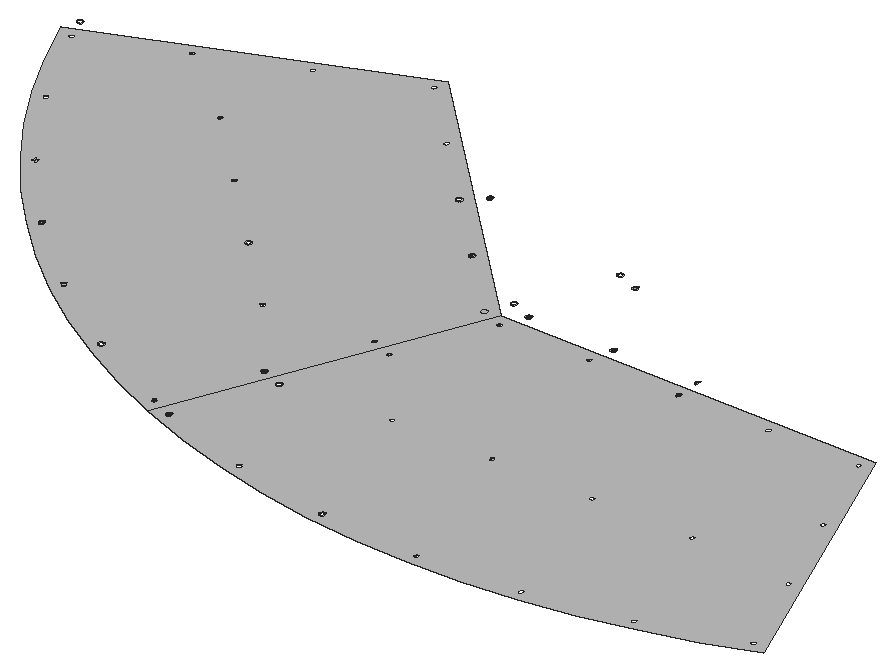
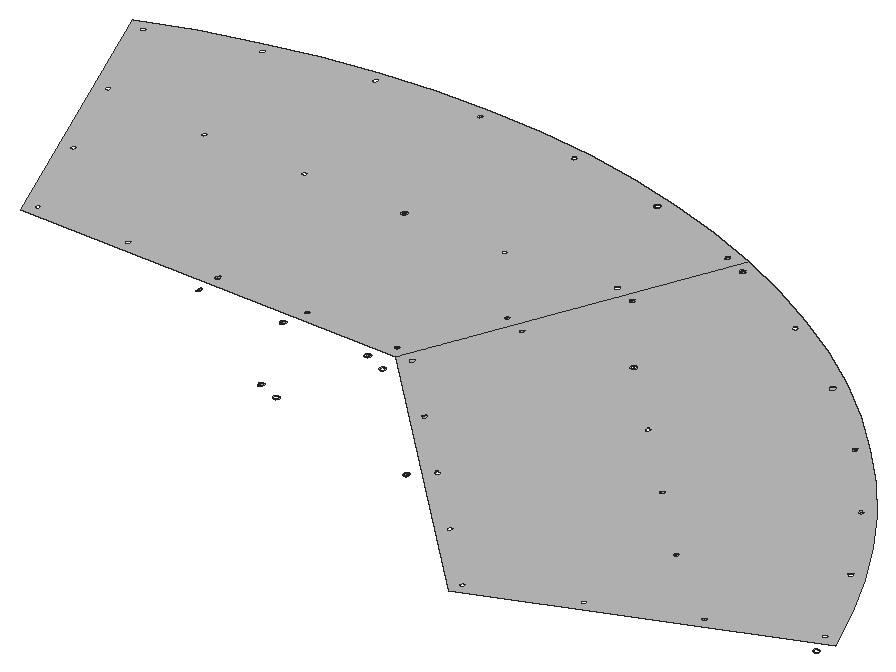
# SketchUp Ruby script. Lengths in inches.
U = 1.inch
M = Sketchup.active_model
def pt(a) = Geom::Point3d.new(a.map { |v| v * U })
def face(e, loops, mat)
  f = e.add_face(loops[0].map { |a| pt(a) })
  loops[1..].each { |l| e.add_face(l.map { |a| pt(a) }).erase! }
  f.material = f.back_material = mat if mat
  f
end
# faces: each face lists its corners as indices into pts; further lists are holes
def faces(e, pts, list, mat = nil) = list.each { |f| face(e, (f[0].is_a?(Array) ? f : [f]).map { |l| l.map { |i| pts[i] } }, mat) }
# xy, xz, yz: faces in a plane at the given z, y or x. An outline is a flat list of corners, or four numbers for a rectangle; further outlines are holes
def ring(l) = l.size == 4 ? [[l[0], l[1]], [l[2], l[1]], [l[2], l[3]], [l[0], l[3]]] : l.each_slice(2).to_a
def flat(e, list, mat, &to3) = list.each { |f| face(e, (f[0].is_a?(Array) ? f : [f]).map { |l| ring(l).map { |u, v| to3.(u, v) } }, mat) }
def xy(e, z, list, mat = nil) = flat(e, list, mat) { |x, y| [x, y, z] }
def xz(e, y, list, mat = nil) = flat(e, list, mat) { |x, z| [x, y, z] }
def yz(e, x, list, mat = nil) = flat(e, list, mat) { |y, z| [x, y, z] }
def lines(e, pts, list) = list.each { |a, b| e.add_line(pt(pts[a]), pt(pts[b])) }
# prism: a flat outline (further loops are holes) pulled along v
def prism(e, loops, v, mat = nil)
  f = face(e, loops, mat); d = Geom::Vector3d.new(v.map { |x| x * U })
  f.pushpull(f.normal.samedirection?(d) ? d.length : -d.length)
end
def box(e, o, s, mat = nil) = prism(e, [[o, [o[0] + s[0], o[1], o[2]], [o[0] + s[0], o[1] + s[1], o[2]], [o[0], o[1] + s[1], o[2]]]], [0, 0, s[2]], mat)
def at(x, y, z, deg = 0) = Geom::Transformation.translation(pt([x, y, z])) * Geom::Transformation.rotation(ORIGIN, Z_AXIS, deg.degrees)
def axes(o, x, y, z) = Geom::Transformation.new([*x, 0, *y, 0, *z, 0, *pt(o).to_a, 1])
def part(name) = M.definitions.add(name)
# library, detail: a bought-in or finely detailed component or shape, given as its bounding box
def library(name, o, s) = part(name).tap { |d| box(d.entities, o, s) }
def detail(e, o, s) = box(e.add_group.entities, o, s)
def put(e, d, t, mat = nil) = e.add_instance(d, t).tap { |i| i.material = mat if mat }
def group(e, t, mat = nil) = e.add_group.tap { |g| g.transformation = t; g.material = mat if mat }.entities
root = M.entities
M.materials.add("[Metal_Steel_Textured_White]").color = [191, 191, 191]
xy(root,3.625,[[[149.818,136.763,148.077,136.82,146.344,136.991,144.626,137.274,142.93,137.67,141.263,138.175,139.633,138.789,143.617,148.407,156.019,148.407,160.003,138.789,158.373,138.175,156.706,137.67,155.01,137.274,153.292,136.991,151.559,136.82],[156.345,137.899,156.368,137.902,156.39,137.911,156.408,137.925,156.422,137.943,156.431,137.965,156.434,137.988,156.431,138.011,156.422,138.032,156.408,138.051,156.39,138.065,156.368,138.074,156.345,138.077,156.322,138.074,156.301,138.065,156.283,138.051,156.269,138.032,156.26,138.011,156.257,137.988,156.26,137.965,156.269,137.943,156.283,137.925,156.301,137.911,156.322,137.902],[143.29,137.899,143.313,137.902,143.335,137.911,143.353,137.925,143.367,137.943,143.376,137.965,143.379,137.988,143.376,138.011,143.367,138.032,143.353,138.051,143.335,138.065,143.313,138.074,143.29,138.077,143.267,138.074,143.246,138.065,143.227,138.051,143.213,138.032,143.204,138.011,143.201,137.988,143.204,137.965,143.213,137.943,143.227,137.925,143.246,137.911,143.267,137.902],[149.818,147.919,149.841,147.922,149.862,147.931,149.881,147.945,149.895,147.963,149.904,147.985,149.907,148.008,149.904,148.031,149.895,148.052,149.881,148.07,149.862,148.085,149.841,148.093,149.818,148.096,149.795,148.093,149.773,148.085,149.755,148.07,149.741,148.052,149.732,148.031,149.729,148.008,149.732,147.985,149.741,147.963,149.755,147.945,149.773,147.931,149.795,147.922],[146.851,147.919,146.874,147.922,146.895,147.931,146.914,147.945,146.928,147.963,146.937,147.985,146.94,148.008,146.937,148.031,146.928,148.052,146.914,148.07,146.895,148.085,146.874,148.093,146.851,148.096,146.828,148.093,146.806,148.085,146.788,148.07,146.774,148.052,146.765,148.031,146.762,148.008,146.765,147.985,146.774,147.963,146.788,147.945,146.806,147.931,146.828,147.922],[152.785,147.919,152.808,147.922,152.829,147.931,152.848,147.945,152.862,147.963,152.871,147.985,152.874,148.008,152.871,148.031,152.862,148.052,152.848,148.07,152.829,148.085,152.808,148.093,152.785,148.096,152.762,148.093,152.741,148.085,152.722,148.07,152.708,148.052,152.699,148.031,152.696,148.008,152.699,147.985,152.708,147.963,152.722,147.945,152.741,147.931,152.762,147.922],[146.528,137.28,146.551,137.283,146.573,137.292,146.591,137.306,146.605,137.325,146.614,137.346,146.617,137.369,146.614,137.392,146.605,137.414,146.591,137.432,146.573,137.446,146.551,137.455,146.528,137.458,146.505,137.455,146.484,137.446,146.465,137.432,146.451,137.414,146.442,137.392,146.439,137.369,146.442,137.346,146.451,137.325,146.465,137.306,146.484,137.292,146.505,137.283],[153.108,137.28,153.131,137.283,153.152,137.292,153.171,137.306,153.185,137.325,153.194,137.346,153.197,137.369,153.194,137.392,153.185,137.414,153.171,137.432,153.152,137.446,153.131,137.455,153.108,137.458,153.085,137.455,153.063,137.446,153.045,137.432,153.031,137.414,153.022,137.392,153.019,137.369,153.022,137.346,153.031,137.325,153.045,137.306,153.063,137.292,153.085,137.283],[158.237,141.919,158.26,141.922,158.282,141.931,158.3,141.945,158.314,141.963,158.323,141.985,158.326,142.008,158.323,142.031,158.314,142.052,158.3,142.07,158.282,142.085,158.26,142.093,158.237,142.096,158.214,142.093,158.193,142.085,158.175,142.07,158.16,142.052,158.152,142.031,158.149,142.008,158.152,141.985,158.16,141.963,158.175,141.945,158.193,141.931,158.214,141.922],[156.995,144.919,157.018,144.922,157.039,144.931,157.058,144.945,157.072,144.963,157.081,144.985,157.084,145.008,157.081,145.031,157.072,145.052,157.058,145.07,157.039,145.085,157.018,145.093,156.995,145.096,156.972,145.093,156.95,145.085,156.932,145.07,156.918,145.052,156.909,145.031,156.906,145.008,156.909,144.985,156.918,144.963,156.932,144.945,156.95,144.931,156.972,144.922],[141.398,141.919,141.421,141.922,141.443,141.931,141.461,141.945,141.475,141.963,141.484,141.985,141.487,142.008,141.484,142.031,141.475,142.052,141.461,142.07,141.443,142.085,141.421,142.093,141.398,142.096,141.375,142.093,141.354,142.085,141.335,142.07,141.321,142.052,141.3125,142.031,141.309,142.008,141.3125,141.985,141.321,141.963,141.335,141.945,141.354,141.931,141.375,141.922],[142.641,144.919,142.664,144.922,142.685,144.931,142.704,144.945,142.718,144.963,142.727,144.985,142.73,145.008,142.727,145.031,142.718,145.052,142.704,145.07,142.685,145.085,142.664,145.093,142.641,145.096,142.618,145.093,142.597,145.085,142.578,145.07,142.564,145.052,142.555,145.031,142.552,145.008,142.555,144.985,142.564,144.963,142.578,144.945,142.597,144.931,142.618,144.922],[155.752,147.919,155.775,147.922,155.797,147.931,155.815,147.945,155.829,147.963,155.838,147.985,155.841,148.008,155.838,148.031,155.829,148.052,155.815,148.07,155.797,148.085,155.775,148.093,155.752,148.096,155.729,148.093,155.708,148.085,155.689,148.07,155.675,148.052,155.666,148.031,155.663,148.008,155.666,147.985,155.675,147.963,155.689,147.945,155.708,147.931,155.729,147.922],[151.473,142.263,151.496,142.266,151.518,142.275,151.536,142.289,151.55,142.307,151.559,142.329,151.562,142.352,151.559,142.375,151.55,142.396,151.536,142.415,151.518,142.429,151.496,142.438,151.473,142.441,151.45,142.438,151.429,142.429,151.41,142.415,151.396,142.396,151.387,142.375,151.384,142.352,151.387,142.329,151.396,142.307,151.41,142.289,151.429,142.275,151.45,142.266],[154.784,142.263,154.807,142.266,154.828,142.275,154.847,142.289,154.861,142.307,154.87,142.329,154.873,142.352,154.87,142.375,154.861,142.396,154.847,142.415,154.828,142.429,154.807,142.438,154.784,142.441,154.761,142.438,154.74,142.429,154.721,142.415,154.707,142.396,154.698,142.375,154.695,142.352,154.698,142.329,154.707,142.307,154.721,142.289,154.74,142.275,154.761,142.266],[148.163,142.263,148.186,142.266,148.207,142.275,148.225,142.289,148.239,142.307,148.248,142.329,148.251,142.352,148.248,142.375,148.239,142.396,148.225,142.415,148.207,142.429,148.186,142.438,148.163,142.441,148.139,142.438,148.118,142.429,148.1,142.415,148.086,142.396,148.077,142.375,148.074,142.352,148.077,142.329,148.086,142.307,148.1,142.289,148.118,142.275,148.139,142.266],[149.818,137.073,149.841,137.076,149.862,137.085,149.881,137.099,149.895,137.118,149.904,137.139,149.907,137.162,149.904,137.185,149.895,137.207,149.881,137.225,149.862,137.239,149.841,137.248,149.818,137.251,149.795,137.248,149.773,137.239,149.755,137.225,149.741,137.207,149.732,137.185,149.729,137.162,149.732,137.139,149.741,137.118,149.755,137.099,149.773,137.085,149.795,137.076],[144.852,142.263,144.875,142.266,144.896,142.275,144.915,142.289,144.929,142.307,144.9375,142.329,144.941,142.352,144.9375,142.375,144.929,142.396,144.915,142.415,144.896,142.429,144.875,142.438,144.852,142.441,144.829,142.438,144.807,142.429,144.789,142.415,144.775,142.396,144.766,142.375,144.763,142.352,144.766,142.329,144.775,142.307,144.789,142.289,144.807,142.275,144.829,142.266],[159.48,138.919,159.503,138.922,159.525,138.931,159.543,138.945,159.557,138.963,159.566,138.985,159.569,139.008,159.566,139.031,159.557,139.052,159.543,139.071,159.525,139.085,159.503,139.094,159.48,139.097,159.457,139.094,159.436,139.085,159.417,139.071,159.403,139.052,159.394,139.031,159.391,139.008,159.394,138.985,159.403,138.963,159.417,138.945,159.436,138.931,159.457,138.922],[140.156,138.919,140.179,138.922,140.2,138.931,140.219,138.945,140.233,138.963,140.242,138.985,140.245,139.008,140.242,139.031,140.233,139.052,140.219,139.071,140.2,139.085,140.179,139.094,140.156,139.097,140.133,139.094,140.111,139.085,140.093,139.071,140.079,139.052,140.07,139.031,140.067,139.008,140.07,138.985,140.079,138.963,140.093,138.945,140.111,138.931,140.133,138.922],[143.884,147.919,143.907,147.922,143.928,147.931,143.946,147.945,143.961,147.963,143.969,147.985,143.972,148.008,143.969,148.031,143.961,148.052,143.946,148.07,143.928,148.085,143.907,148.093,143.884,148.096,143.861,148.093,143.839,148.085,143.821,148.07,143.807,148.052,143.798,148.031,143.795,148.008,143.798,147.985,143.807,147.963,143.821,147.945,143.839,147.931,143.861,147.922]],[149.818,137.142,149.813,137.143,149.808,137.145,149.804,137.148,149.801,137.152,149.799,137.157,149.798,137.162,149.799,137.167,149.801,137.172,149.804,137.176,149.808,137.179,149.813,137.181,149.818,137.182],[[146.528,137.28,146.505,137.283,146.484,137.292,146.465,137.306,146.451,137.325,146.442,137.346,146.439,137.369,146.442,137.392,146.451,137.414,146.465,137.432,146.484,137.446,146.505,137.455,146.528,137.458,146.551,137.455,146.573,137.446,146.591,137.432,146.605,137.414,146.614,137.392,146.617,137.369,146.614,137.346,146.605,137.325,146.591,137.306,146.573,137.292,146.551,137.283],[146.528,137.281,146.551,137.284,146.572,137.293,146.59,137.307,146.604,137.325,146.613,137.347,146.616,137.369,146.613,137.392,146.604,137.413,146.59,137.432,146.572,137.445,146.551,137.454,146.528,137.457,146.505,137.454,146.484,137.445,146.466,137.432,146.452,137.413,146.443,137.392,146.44,137.369,146.443,137.347,146.452,137.325,146.466,137.307,146.484,137.293,146.505,137.284]],[[143.29,137.899,143.267,137.902,143.246,137.911,143.227,137.925,143.213,137.943,143.204,137.965,143.201,137.988,143.204,138.011,143.213,138.032,143.227,138.051,143.246,138.065,143.267,138.074,143.29,138.077,143.313,138.074,143.335,138.065,143.353,138.051,143.367,138.032,143.376,138.011,143.379,137.988,143.376,137.965,143.367,137.943,143.353,137.925,143.335,137.911,143.313,137.902],[143.29,137.9,143.313,137.903,143.334,137.912,143.352,137.926,143.366,137.944,143.375,137.965,143.378,137.988,143.375,138.011,143.366,138.032,143.352,138.05,143.334,138.064,143.313,138.073,143.29,138.076,143.268,138.073,143.246,138.064,143.228,138.05,143.214,138.032,143.205,138.011,143.202,137.988,143.205,137.965,143.214,137.944,143.228,137.926,143.246,137.912,143.268,137.903]],[[139.633,138.789,138.047,139.508,136.511,140.329,135.032,141.248,133.616,142.263,132.27,143.368,130.999,144.558,129.808,145.829,128.703,147.176,127.689,148.591,126.769,150.07,125.948,151.606,125.229,153.192,134.847,157.176,143.617,148.407],[127.249,149.951,127.272,149.954,127.293,149.963,127.312,149.977,127.326,149.995,127.335,150.017,127.338,150.04,127.335,150.063,127.326,150.084,127.312,150.103,127.293,150.117,127.272,150.126,127.249,150.129,127.226,150.126,127.205,150.117,127.186,150.103,127.172,150.084,127.163,150.063,127.16,150.04,127.163,150.017,127.172,149.995,127.186,149.977,127.205,149.963,127.226,149.954],[141.903,145.224,141.926,145.227,141.948,145.236,141.966,145.25,141.98,145.269,141.989,145.29,141.992,145.313,141.989,145.336,141.98,145.358,141.966,145.376,141.948,145.39,141.926,145.399,141.903,145.402,141.88,145.399,141.859,145.39,141.84,145.376,141.826,145.358,141.817,145.336,141.814,145.313,141.817,145.29,141.826,145.269,141.84,145.25,141.859,145.236,141.88,145.227],[136.48,140.72,136.503,140.723,136.525,140.732,136.543,140.746,136.557,140.764,136.566,140.786,136.569,140.809,136.566,140.832,136.557,140.853,136.543,140.871,136.525,140.886,136.503,140.894,136.48,140.897,136.457,140.894,136.436,140.886,136.418,140.871,136.403,140.853,136.395,140.832,136.392,140.809,136.395,140.786,136.403,140.764,136.418,140.746,136.436,140.732,136.457,140.723],[141.048,150.322,141.071,150.325,141.092,150.334,141.111,150.348,141.125,150.367,141.134,150.388,141.137,150.411,141.134,150.434,141.125,150.456,141.111,150.474,141.092,150.488,141.071,150.497,141.048,150.5,141.025,150.497,141.003,150.488,140.985,150.474,140.971,150.456,140.962,150.434,140.959,150.411,140.962,150.388,140.971,150.367,140.985,150.348,141.003,150.334,141.025,150.325],[139.418,139.224,139.441,139.227,139.462,139.236,139.481,139.25,139.495,139.269,139.504,139.29,139.507,139.313,139.504,139.336,139.495,139.358,139.481,139.376,139.462,139.39,139.441,139.399,139.418,139.402,139.395,139.399,139.374,139.39,139.355,139.376,139.341,139.358,139.332,139.336,139.329,139.313,139.332,139.29,139.341,139.269,139.355,139.25,139.374,139.236,139.395,139.227],[140.661,142.224,140.684,142.227,140.705,142.236,140.724,142.25,140.738,142.269,140.747,142.29,140.75,142.313,140.747,142.336,140.738,142.358,140.724,142.376,140.705,142.39,140.684,142.399,140.661,142.402,140.638,142.399,140.616,142.39,140.598,142.376,140.584,142.358,140.575,142.336,140.572,142.313,140.575,142.29,140.584,142.269,140.598,142.25,140.616,142.236,140.638,142.227],[129.101,147.224,129.124,147.227,129.146,147.236,129.164,147.25,129.178,147.269,129.187,147.29,129.19,147.313,129.187,147.336,129.178,147.358,129.164,147.376,129.146,147.39,129.124,147.399,129.101,147.402,129.078,147.399,129.057,147.39,129.038,147.376,129.024,147.358,129.015,147.336,129.012,147.313,129.015,147.29,129.024,147.269,129.038,147.25,129.057,147.236,129.078,147.227],[133.78,149.592,133.803,149.595,133.825,149.604,133.843,149.618,133.857,149.636,133.866,149.658,133.869,149.681,133.866,149.704,133.857,149.725,133.843,149.744,133.825,149.758,133.803,149.767,133.78,149.77,133.757,149.767,133.736,149.758,133.717,149.744,133.703,149.725,133.694,149.704,133.691,149.681,133.694,149.658,133.703,149.636,133.717,149.618,133.736,149.604,133.757,149.595],[133.754,142.572,133.777,142.575,133.798,142.584,133.816,142.598,133.831,142.616,133.839,142.638,133.843,142.661,133.839,142.684,133.831,142.705,133.816,142.724,133.798,142.738,133.777,142.747,133.754,142.75,133.731,142.747,133.709,142.738,133.691,142.724,133.677,142.705,133.668,142.684,133.665,142.661,133.668,142.638,133.677,142.616,133.691,142.598,133.709,142.584,133.731,142.575],[138.462,144.91,138.485,144.913,138.507,144.922,138.525,144.936,138.539,144.954,138.548,144.976,138.551,144.999,138.548,145.022,138.539,145.043,138.525,145.061,138.507,145.076,138.485,145.084,138.462,145.087,138.439,145.084,138.418,145.076,138.399,145.061,138.385,145.043,138.376,145.022,138.373,144.999,138.376,144.976,138.385,144.954,138.399,144.936,138.418,144.922,138.439,144.913],[131.754,155.374,131.777,155.377,131.798,155.386,131.816,155.4,131.831,155.418,131.839,155.44,131.842,155.463,131.839,155.486,131.831,155.507,131.816,155.526,131.798,155.54,131.777,155.549,131.754,155.552,131.731,155.549,131.709,155.54,131.691,155.526,131.677,155.507,131.668,155.486,131.665,155.463,131.668,155.44,131.677,155.418,131.691,155.4,131.709,155.386,131.731,155.377],[136.852,154.518,136.875,154.521,136.896,154.53,136.914,154.545,136.929,154.563,136.9375,154.584,136.941,154.607,136.9375,154.63,136.929,154.652,136.914,154.67,136.896,154.684,136.875,154.693,136.852,154.696,136.829,154.693,136.807,154.684,136.789,154.67,136.775,154.652,136.766,154.63,136.763,154.607,136.766,154.584,136.775,154.563,136.789,154.545,136.807,154.53,136.829,154.521],[138.95,152.42,138.973,152.423,138.994,152.432,139.013,152.446,139.027,152.465,139.036,152.486,139.039,152.509,139.036,152.532,139.027,152.554,139.013,152.572,138.994,152.586,138.973,152.595,138.95,152.598,138.927,152.595,138.905,152.586,138.887,152.572,138.873,152.554,138.864,152.532,138.861,152.509,138.864,152.486,138.873,152.465,138.887,152.446,138.905,152.432,138.927,152.423],[131.439,151.933,131.462,151.936,131.483,151.945,131.502,151.959,131.516,151.977,131.525,151.999,131.528,152.022,131.525,152.045,131.516,152.066,131.502,152.085,131.483,152.099,131.462,152.108,131.439,152.111,131.416,152.108,131.395,152.099,131.376,152.085,131.362,152.066,131.353,152.045,131.35,152.022,131.353,151.999,131.362,151.977,131.376,151.959,131.395,151.945,131.416,151.936],[131.281,144.751,131.304,144.755,131.325,144.763,131.344,144.778,131.358,144.796,131.367,144.817,131.37,144.84,131.367,144.863,131.358,144.885,131.344,144.903,131.325,144.917,131.304,144.926,131.281,144.929,131.258,144.926,131.236,144.917,131.218,144.903,131.204,144.885,131.195,144.863,131.192,144.84,131.195,144.817,131.204,144.796,131.218,144.778,131.236,144.763,131.258,144.755],[125.754,152.889,125.777,152.892,125.798,152.901,125.817,152.915,125.831,152.933,125.84,152.955,125.843,152.978,125.84,153.001,125.831,153.022,125.817,153.04,125.798,153.055,125.777,153.063,125.754,153.066,125.731,153.063,125.709,153.055,125.691,153.04,125.677,153.022,125.668,153.001,125.665,152.978,125.668,152.955,125.677,152.933,125.691,152.915,125.709,152.901,125.731,152.892],[143.146,148.224,143.169,148.227,143.19,148.236,143.209,148.25,143.223,148.269,143.232,148.29,143.235,148.313,143.232,148.336,143.223,148.358,143.209,148.376,143.19,148.39,143.169,148.399,143.146,148.402,143.123,148.399,143.101,148.39,143.083,148.376,143.069,148.358,143.06,148.336,143.057,148.313,143.06,148.29,143.069,148.269,143.083,148.25,143.101,148.236,143.123,148.227],[134.754,156.617,134.777,156.62,134.798,156.628,134.816,156.643,134.831,156.661,134.839,156.682,134.842,156.705,134.839,156.728,134.831,156.75,134.816,156.768,134.798,156.782,134.777,156.791,134.754,156.794,134.731,156.791,134.709,156.782,134.691,156.768,134.677,156.75,134.668,156.728,134.665,156.705,134.668,156.682,134.677,156.661,134.691,156.643,134.709,156.628,134.731,156.62],[128.754,154.131,128.777,154.134,128.798,154.143,128.816,154.157,128.831,154.176,128.839,154.197,128.843,154.22,128.839,154.243,128.831,154.265,128.816,154.283,128.798,154.297,128.777,154.306,128.754,154.309,128.731,154.306,128.709,154.297,128.691,154.283,128.677,154.265,128.668,154.243,128.665,154.22,128.668,154.197,128.677,154.176,128.691,154.157,128.709,154.143,128.731,154.134],[136.121,147.251,136.144,147.254,136.166,147.263,136.184,147.277,136.198,147.295,136.207,147.317,136.21,147.34,136.207,147.363,136.198,147.384,136.184,147.402,136.166,147.417,136.144,147.425,136.121,147.429,136.098,147.425,136.077,147.417,136.058,147.402,136.044,147.384,136.035,147.363,136.032,147.34,136.035,147.317,136.044,147.295,136.058,147.277,136.077,147.263,136.098,147.254]],
  [[140.156,138.919,140.133,138.922,140.111,138.931,140.093,138.945,140.079,138.963,140.07,138.985,140.067,139.008,140.07,139.031,140.079,139.052,140.093,139.071,140.111,139.085,140.133,139.094,140.156,139.097,140.179,139.094,140.2,139.085,140.219,139.071,140.233,139.052,140.242,139.031,140.245,139.008,140.242,138.985,140.233,138.963,140.219,138.945,140.2,138.931,140.179,138.922],[140.156,138.92,140.178,138.923,140.2,138.932,140.218,138.945,140.232,138.964,140.241,138.985,140.244,139.008,140.241,139.03,140.232,139.052,140.218,139.07,140.2,139.084,140.178,139.093,140.156,139.096,140.133,139.093,140.112,139.084,140.094,139.07,140.08,139.052,140.071,139.03,140.068,139.008,140.071,138.985,140.08,138.964,140.094,138.945,140.112,138.932,140.133,138.923]],[[140.156,138.971,140.146,138.972,140.137,138.976,140.13,138.982,140.124,138.989,140.12,138.998,140.119,139.008,140.12,139.017,140.124,139.026,140.13,139.034,140.137,139.039,140.146,139.043,140.156,139.044,140.165,139.043,140.174,139.039,140.182,139.034,140.1875,139.026,140.191,139.017,140.192,139.008,140.191,138.998,140.1875,138.989,140.182,138.982,140.174,138.976,140.165,138.972],[140.151,138.988,140.161,138.988,140.166,138.99,140.17,138.994,140.173,138.998,140.175,139.002,140.176,139.008,140.175,139.013,140.173,139.018,140.17,139.022,140.166,139.025,140.161,139.027,140.156,139.028,140.151,139.027,140.146,139.025,140.142,139.022,140.138,139.018,140.136,139.013,140.136,139.002,140.138,138.998,140.146,138.99]],[140.151,138.988,140.146,138.99,140.138,138.998,140.136,139.002,140.136,139.013,140.138,139.018,140.142,139.022,140.146,139.025,140.151,139.027,140.156,139.028,140.161,139.027,140.166,139.025,140.17,139.022,140.173,139.018,140.175,139.013,140.176,139.008,140.175,139.002,140.173,138.998,140.17,138.994,140.166,138.99,140.161,138.988],[[139.418,139.224,139.395,139.227,139.374,139.236,139.355,139.25,139.341,139.269,139.332,139.29,139.329,139.313,139.332,139.336,139.341,139.358,139.355,139.376,139.374,139.39,139.395,139.399,139.418,139.402,139.441,139.399,139.462,139.39,139.481,139.376,139.495,139.358,139.504,139.336,139.507,139.313,139.504,139.29,139.495,139.269,139.481,139.25,139.462,139.236,139.441,139.227],[139.418,139.225,139.441,139.228,139.462,139.237,139.48,139.251,139.494,139.269,139.503,139.29,139.506,139.313,139.503,139.336,139.494,139.357,139.48,139.375,139.462,139.389,139.441,139.398,139.418,139.401,139.395,139.398,139.374,139.389,139.356,139.375,139.342,139.357,139.333,139.336,139.33,139.313,139.333,139.29,139.342,139.269,139.356,139.251,139.374,139.237,139.395,139.228]],[[139.418,139.277,139.409,139.278,139.4,139.282,139.392,139.287,139.386,139.295,139.383,139.304,139.381,139.313,139.383,139.323,139.386,139.331,139.392,139.339,139.4,139.345,139.409,139.349,139.418,139.35,139.428,139.349,139.436,139.345,139.444,139.339,139.45,139.331,139.453,139.323,139.455,139.313,139.453,139.304,139.45,139.295,139.444,139.287,139.436,139.282,139.428,139.278],[139.418,139.293,139.423,139.294,139.428,139.296,139.432,139.299,139.435,139.303,139.4375,139.308,139.438,139.313,139.4375,139.318,139.435,139.323,139.432,139.327,139.428,139.33,139.423,139.332,139.418,139.333,139.413,139.332,139.408,139.33,139.404,139.327,139.401,139.323,139.399,139.318,139.398,139.313,139.399,139.308,139.401,139.303,139.404,139.299,139.408,139.296,139.413,139.294]],
  [139.418,139.293,139.413,139.294,139.408,139.296,139.404,139.299,139.401,139.303,139.399,139.308,139.398,139.313,139.399,139.318,139.401,139.323,139.404,139.327,139.408,139.33,139.413,139.332,139.418,139.333,139.423,139.332,139.428,139.33,139.432,139.327,139.435,139.323,139.4375,139.318,139.438,139.313,139.4375,139.308,139.435,139.303,139.432,139.299,139.428,139.296,139.423,139.294],[[136.48,140.72,136.457,140.723,136.436,140.732,136.418,140.746,136.403,140.764,136.395,140.786,136.392,140.809,136.395,140.832,136.403,140.853,136.418,140.871,136.436,140.886,136.457,140.894,136.48,140.897,136.503,140.894,136.525,140.886,136.543,140.871,136.557,140.853,136.566,140.832,136.569,140.809,136.566,140.786,136.557,140.764,136.543,140.746,136.525,140.732,136.503,140.723],[136.48,140.721,136.503,140.724,136.524,140.732,136.543,140.746,136.557,140.765,136.565,140.786,136.568,140.809,136.565,140.831,136.557,140.852,136.543,140.871,136.524,140.885,136.503,140.893,136.48,140.896,136.458,140.893,136.436,140.885,136.418,140.871,136.404,140.852,136.395,140.831,136.392,140.809,136.395,140.786,136.404,140.765,136.418,140.746,136.436,140.732,136.458,140.724]],[[141.398,141.919,141.375,141.922,141.354,141.931,141.335,141.945,141.321,141.963,141.3125,141.985,141.309,142.008,141.3125,142.031,141.321,142.052,141.335,142.07,141.354,142.085,141.375,142.093,141.398,142.096,141.421,142.093,141.443,142.085,141.461,142.07,141.475,142.052,141.484,142.031,141.487,142.008,141.484,141.985,141.475,141.963,141.461,141.945,141.443,141.931,141.421,141.922],[141.398,141.92,141.421,141.923,141.442,141.931,141.461,141.945,141.474,141.964,141.483,141.985,141.486,142.008,141.483,142.03,141.474,142.052,141.461,142.07,141.442,142.084,141.421,142.093,141.398,142.096,141.376,142.093,141.354,142.084,141.336,142.07,141.322,142.052,141.313,142.03,141.31,142.008,141.313,141.985,141.322,141.964,141.336,141.945,141.354,141.931,141.376,141.923]],[[140.661,142.224,140.638,142.227,140.616,142.236,140.598,142.25,140.584,142.269,140.575,142.29,140.572,142.313,140.575,142.336,140.584,142.358,140.598,142.376,140.616,142.39,140.638,142.399,140.661,142.402,140.684,142.399,140.705,142.39,140.724,142.376,140.738,142.358,140.747,142.336,140.75,142.313,140.747,142.29,140.738,142.269,140.724,142.25,140.705,142.236,140.684,142.227],[140.661,142.225,140.683,142.228,140.705,142.237,140.723,142.251,140.737,142.269,140.746,142.29,140.749,142.313,140.746,142.336,140.737,142.357,140.723,142.375,140.705,142.389,140.683,142.398,140.661,142.401,140.638,142.398,140.617,142.389,140.599,142.375,140.585,142.357,140.576,142.336,140.573,142.313,140.576,142.29,140.585,142.269,140.599,142.251,140.617,142.237,140.638,142.228]],[[148.163,142.263,148.139,142.266,148.118,142.275,148.1,142.289,148.086,142.307,148.077,142.329,148.074,142.352,148.077,142.375,148.086,142.396,148.1,142.415,148.118,142.429,148.139,142.438,148.163,142.441,148.186,142.438,148.207,142.429,148.225,142.415,148.239,142.396,148.248,142.375,148.251,142.352,148.248,142.329,148.239,142.307,148.225,142.289,148.207,142.275,148.186,142.266],[148.163,142.264,148.185,142.267,148.206,142.276,148.225,142.29,148.239,142.308,148.247,142.329,148.25,142.352,148.247,142.375,148.239,142.396,148.225,142.414,148.206,142.428,148.185,142.437,148.163,142.44,148.14,142.437,148.119,142.428,148.1,142.414,148.086,142.396,148.078,142.375,148.075,142.352,148.078,142.329,148.086,142.308,148.1,142.29,148.119,142.276,148.14,142.267]],
  [[140.661,142.277,140.651,142.278,140.642,142.281,140.635,142.287,140.629,142.295,140.625,142.304,140.624,142.313,140.625,142.323,140.629,142.331,140.635,142.339,140.642,142.345,140.651,142.349,140.661,142.35,140.67,142.349,140.679,142.345,140.687,142.339,140.692,142.331,140.696,142.323,140.697,142.313,140.696,142.304,140.692,142.295,140.687,142.287,140.679,142.281,140.67,142.278],[140.661,142.293,140.666,142.294,140.671,142.296,140.675,142.299,140.678,142.303,140.68,142.308,140.681,142.313,140.68,142.318,140.678,142.323,140.675,142.327,140.671,142.33,140.666,142.332,140.661,142.333,140.656,142.332,140.651,142.33,140.647,142.327,140.643,142.323,140.641,142.318,140.641,142.308,140.643,142.303,140.647,142.299,140.651,142.296,140.656,142.294]],[140.661,142.293,140.656,142.294,140.651,142.296,140.647,142.299,140.643,142.303,140.641,142.308,140.641,142.318,140.643,142.323,140.647,142.327,140.651,142.33,140.656,142.332,140.661,142.333,140.666,142.332,140.671,142.33,140.675,142.327,140.678,142.323,140.68,142.318,140.681,142.313,140.68,142.308,140.678,142.303,140.675,142.299,140.671,142.296,140.666,142.294],[[148.163,142.315,148.153,142.317,148.144,142.32,148.137,142.326,148.131,142.334,148.127,142.342,148.126,142.352,148.127,142.361,148.131,142.37,148.137,142.378,148.144,142.384,148.153,142.387,148.163,142.389,148.172,142.387,148.181,142.384,148.188,142.378,148.194,142.37,148.198,142.361,148.199,142.352,148.198,142.342,148.194,142.334,148.188,142.326,148.181,142.32,148.172,142.317],[148.163,142.332,148.168,142.333,148.172,142.335,148.177,142.338,148.18,142.342,148.182,142.347,148.182,142.357,148.18,142.362,148.177,142.366,148.172,142.369,148.168,142.371,148.163,142.372,148.157,142.371,148.153,142.369,148.148,142.366,148.145,142.362,148.143,142.357,148.143,142.347,148.145,142.342,148.148,142.338,148.153,142.335,148.157,142.333]],[148.163,142.332,148.157,142.333,148.153,142.335,148.148,142.338,148.145,142.342,148.143,142.347,148.143,142.357,148.145,142.362,148.148,142.366,148.153,142.369,148.157,142.371,148.163,142.372,148.168,142.371,148.172,142.369,148.177,142.366,148.18,142.362,148.182,142.357,148.182,142.347,148.18,142.342,148.177,142.338,148.172,142.335,148.168,142.333],[[133.754,142.572,133.731,142.575,133.709,142.584,133.691,142.598,133.677,142.616,133.668,142.638,133.665,142.661,133.668,142.684,133.677,142.705,133.691,142.724,133.709,142.738,133.731,142.747,133.754,142.75,133.777,142.747,133.798,142.738,133.816,142.724,133.831,142.705,133.839,142.684,133.843,142.661,133.839,142.638,133.831,142.616,133.816,142.598,133.798,142.584,133.777,142.575],[133.754,142.573,133.776,142.576,133.798,142.585,133.816,142.599,133.83,142.617,133.839,142.638,133.842,142.661,133.839,142.683,133.83,142.705,133.816,142.723,133.798,142.737,133.776,142.746,133.754,142.749,133.731,142.746,133.71,142.737,133.691,142.723,133.677,142.705,133.669,142.683,133.666,142.661,133.669,142.638,133.677,142.617,133.691,142.599,133.71,142.585,133.731,142.576]],
  [[133.754,142.573,133.731,142.576,133.71,142.585,133.691,142.599,133.677,142.617,133.669,142.638,133.666,142.661,133.669,142.683,133.677,142.705,133.691,142.723,133.71,142.737,133.731,142.746,133.754,142.749,133.776,142.746,133.798,142.737,133.816,142.723,133.83,142.705,133.839,142.683,133.842,142.661,133.839,142.638,133.83,142.617,133.816,142.599,133.798,142.585,133.776,142.576],[133.754,142.624,133.763,142.625,133.772,142.629,133.78,142.635,133.785,142.642,133.789,142.651,133.79,142.661,133.789,142.67,133.785,142.679,133.78,142.687,133.772,142.692,133.763,142.696,133.754,142.697,133.744,142.696,133.735,142.692,133.728,142.687,133.722,142.679,133.718,142.67,133.717,142.661,133.718,142.651,133.722,142.642,133.728,142.635,133.735,142.629,133.744,142.625]],[[131.281,144.751,131.258,144.755,131.236,144.763,131.218,144.778,131.204,144.796,131.195,144.817,131.192,144.84,131.195,144.863,131.204,144.885,131.218,144.903,131.236,144.917,131.258,144.926,131.281,144.929,131.304,144.926,131.325,144.917,131.344,144.903,131.358,144.885,131.367,144.863,131.37,144.84,131.367,144.817,131.358,144.796,131.344,144.778,131.325,144.763,131.304,144.755],[131.281,144.752,131.304,144.755,131.325,144.764,131.343,144.778,131.357,144.796,131.366,144.818,131.369,144.84,131.366,144.863,131.357,144.884,131.343,144.903,131.325,144.917,131.304,144.925,131.281,144.928,131.258,144.925,131.237,144.917,131.219,144.903,131.205,144.884,131.196,144.863,131.193,144.84,131.196,144.818,131.205,144.796,131.219,144.778,131.237,144.764,131.258,144.755]],[[131.281,144.804,131.271,144.805,131.263,144.809,131.255,144.815,131.249,144.822,131.246,144.831,131.244,144.84,131.246,144.85,131.249,144.859,131.255,144.866,131.263,144.872,131.271,144.876,131.281,144.877,131.29,144.876,131.299,144.872,131.307,144.866,131.3125,144.859,131.316,144.85,131.317,144.84,131.316,144.831,131.3125,144.822,131.307,144.815,131.299,144.809,131.29,144.805],[131.281,144.82,131.286,144.821,131.291,144.823,131.295,144.826,131.298,144.83,131.3,144.835,131.301,144.84,131.3,144.846,131.298,144.85,131.295,144.854,131.291,144.858,131.286,144.86,131.276,144.86,131.271,144.858,131.267,144.854,131.264,144.85,131.262,144.846,131.261,144.84,131.262,144.835,131.264,144.83,131.267,144.826,131.271,144.823,131.276,144.821]],[131.281,144.82,131.276,144.821,131.271,144.823,131.267,144.826,131.264,144.83,131.262,144.835,131.261,144.84,131.262,144.846,131.264,144.85,131.267,144.854,131.271,144.858,131.276,144.86,131.286,144.86,131.291,144.858,131.295,144.854,131.298,144.85,131.3,144.846,131.301,144.84,131.3,144.835,131.298,144.83,131.295,144.826,131.291,144.823,131.286,144.821],[[138.462,144.91,138.439,144.913,138.418,144.922,138.399,144.936,138.385,144.954,138.376,144.976,138.373,144.999,138.376,145.022,138.385,145.043,138.399,145.061,138.418,145.076,138.439,145.084,138.462,145.087,138.485,145.084,138.507,145.076,138.525,145.061,138.539,145.043,138.548,145.022,138.551,144.999,138.548,144.976,138.539,144.954,138.525,144.936,138.507,144.922,138.485,144.913],[138.462,144.911,138.485,144.914,138.506,144.922,138.524,144.936,138.538,144.955,138.547,144.976,138.55,144.999,138.547,145.021,138.538,145.043,138.524,145.061,138.506,145.075,138.485,145.083,138.462,145.086,138.439,145.083,138.418,145.075,138.4,145.061,138.386,145.043,138.377,145.021,138.374,144.999,138.377,144.976,138.386,144.955,138.4,144.936,138.418,144.922,138.439,144.914]],
  [[142.641,144.971,142.631,144.972,142.623,144.976,142.615,144.982,142.609,144.989,142.606,144.998,142.604,145.008,142.606,145.017,142.609,145.026,142.615,145.033,142.623,145.039,142.631,145.043,142.641,145.044,142.65,145.043,142.659,145.039,142.667,145.033,142.673,145.026,142.676,145.017,142.678,145.008,142.676,144.998,142.673,144.989,142.667,144.982,142.659,144.976,142.65,144.972],[142.636,144.988,142.646,144.988,142.651,144.99,142.655,144.993,142.658,144.998,142.66,145.002,142.661,145.008,142.66,145.013,142.658,145.018,142.655,145.022,142.651,145.025,142.646,145.027,142.641,145.028,142.636,145.027,142.631,145.025,142.627,145.022,142.624,145.018,142.622,145.013,142.621,145.008,142.622,145.002,142.624,144.998,142.627,144.993,142.631,144.99]],[138.457,144.979,138.452,144.981,138.448,144.984,138.445,144.989,138.443,144.993,138.442,144.999,138.443,145.004,138.445,145.009,138.448,145.013,138.452,145.016,138.457,145.018,138.462,145.019,138.467,145.018,138.472,145.016,138.476,145.013,138.48,145.009,138.482,145.004,138.482,144.993,138.48,144.989,138.476,144.984,138.472,144.981,138.467,144.979],[142.636,144.988,142.631,144.99,142.627,144.993,142.624,144.998,142.622,145.002,142.621,145.008,142.622,145.013,142.624,145.018,142.627,145.022,142.631,145.025,142.636,145.027,142.641,145.028,142.646,145.027,142.651,145.025,142.655,145.022,142.658,145.018,142.66,145.013,142.661,145.008,142.66,145.002,142.658,144.998,142.655,144.993,142.651,144.99,142.646,144.988],[[141.903,145.277,141.894,145.278,141.885,145.281,141.877,145.287,141.872,145.295,141.868,145.304,141.867,145.313,141.868,145.323,141.872,145.331,141.877,145.339,141.885,145.345,141.894,145.348,141.903,145.35,141.913,145.348,141.922,145.345,141.929,145.339,141.935,145.331,141.939,145.323,141.94,145.313,141.939,145.304,141.935,145.295,141.929,145.287,141.922,145.281,141.913,145.278],[141.903,145.293,141.908,145.294,141.913,145.296,141.917,145.299,141.921,145.303,141.923,145.308,141.923,145.318,141.921,145.323,141.917,145.327,141.913,145.33,141.908,145.332,141.903,145.333,141.898,145.332,141.893,145.33,141.889,145.327,141.886,145.323,141.884,145.318,141.883,145.313,141.884,145.308,141.886,145.303,141.889,145.299,141.893,145.296,141.898,145.294]],[141.903,145.293,141.898,145.294,141.893,145.296,141.889,145.299,141.886,145.303,141.884,145.308,141.883,145.313,141.884,145.318,141.886,145.323,141.889,145.327,141.893,145.33,141.898,145.332,141.903,145.333,141.908,145.332,141.913,145.33,141.917,145.327,141.921,145.323,141.923,145.318,141.923,145.308,141.921,145.303,141.917,145.299,141.913,145.296,141.908,145.294],
  [[129.101,147.225,129.078,147.228,129.057,147.237,129.039,147.251,129.025,147.269,129.016,147.29,129.013,147.313,129.016,147.336,129.025,147.357,129.039,147.375,129.057,147.389,129.078,147.398,129.101,147.401,129.124,147.398,129.145,147.389,129.163,147.375,129.177,147.357,129.186,147.336,129.189,147.313,129.186,147.29,129.177,147.269,129.163,147.251,129.145,147.237,129.124,147.228],[129.101,147.277,129.111,147.278,129.119,147.281,129.127,147.287,129.133,147.295,129.137,147.304,129.138,147.313,129.137,147.323,129.133,147.331,129.127,147.339,129.119,147.345,129.111,147.349,129.101,147.35,129.092,147.349,129.083,147.345,129.075,147.339,129.069,147.331,129.066,147.323,129.065,147.313,129.066,147.304,129.069,147.295,129.075,147.287,129.083,147.281,129.092,147.278]],[[136.121,147.251,136.098,147.254,136.077,147.263,136.058,147.277,136.044,147.295,136.035,147.317,136.032,147.34,136.035,147.363,136.044,147.384,136.058,147.402,136.077,147.417,136.098,147.425,136.121,147.429,136.144,147.425,136.166,147.417,136.184,147.402,136.198,147.384,136.207,147.363,136.21,147.34,136.207,147.317,136.198,147.295,136.184,147.277,136.166,147.263,136.144,147.254],[136.121,147.252,136.144,147.255,136.165,147.263,136.183,147.277,136.197,147.296,136.206,147.317,136.209,147.34,136.206,147.362,136.197,147.384,136.183,147.402,136.165,147.416,136.144,147.425,136.121,147.428,136.098,147.425,136.077,147.416,136.059,147.402,136.045,147.384,136.036,147.362,136.033,147.34,136.036,147.317,136.045,147.296,136.059,147.277,136.077,147.263,136.098,147.255]],[149.818,147.919,149.795,147.922,149.773,147.931,149.755,147.945,149.741,147.963,149.732,147.985,149.729,148.008,149.732,148.031,149.741,148.052,149.755,148.07,149.773,148.085,149.795,148.093,149.818,148.096,149.818,148.095,149.795,148.092,149.774,148.084,149.756,148.07,149.742,148.051,149.733,148.03,149.73,148.008,149.733,147.985,149.742,147.964,149.756,147.945,149.774,147.931,149.795,147.923,149.818,147.92],[[149.818,147.92,149.795,147.923,149.774,147.931,149.756,147.945,149.742,147.964,149.733,147.985,149.73,148.008,149.733,148.03,149.742,148.051,149.756,148.07,149.774,148.084,149.795,148.092,149.818,148.095,149.818,148.044,149.827,148.043,149.836,148.039,149.844,148.033,149.85,148.026,149.853,148.017,149.854,148.008,149.853,147.998,149.85,147.989,149.844,147.982,149.836,147.976,149.827,147.972,149.818,147.971],[149.813,147.988,149.823,147.988,149.828,147.99,149.832,147.993,149.835,147.998,149.837,148.002,149.838,148.008,149.837,148.013,149.835,148.018,149.832,148.022,149.828,148.025,149.823,148.027,149.813,148.027,149.808,148.025,149.804,148.022,149.801,148.018,149.799,148.013,149.798,148.008,149.799,148.002,149.801,147.998,149.804,147.993,149.808,147.99]],[[143.884,147.971,143.874,147.972,143.865,147.976,143.858,147.982,143.852,147.989,143.848,147.998,143.847,148.008,143.848,148.017,143.852,148.026,143.858,148.033,143.865,148.039,143.874,148.043,143.884,148.044,143.893,148.043,143.902,148.039,143.909,148.033,143.915,148.026,143.919,148.017,143.92,148.008,143.919,147.998,143.915,147.989,143.909,147.982,143.902,147.976,143.893,147.972],[143.878,147.988,143.889,147.988,143.894,147.99,143.898,147.993,143.901,147.998,143.903,148.002,143.904,148.008,143.903,148.013,143.901,148.018,143.898,148.022,143.894,148.025,143.889,148.027,143.878,148.027,143.874,148.025,143.869,148.022,143.866,148.018,143.864,148.013,143.864,148.002,143.866,147.998,143.869,147.993,143.874,147.99]],
  [[146.851,147.971,146.841,147.972,146.832,147.976,146.825,147.982,146.819,147.989,146.815,147.998,146.814,148.008,146.815,148.017,146.819,148.026,146.825,148.033,146.832,148.039,146.841,148.043,146.851,148.044,146.86,148.043,146.869,148.039,146.877,148.033,146.882,148.026,146.886,148.017,146.887,148.008,146.886,147.998,146.882,147.989,146.877,147.982,146.869,147.976,146.86,147.972],[146.846,147.988,146.856,147.988,146.861,147.99,146.865,147.993,146.868,147.998,146.87,148.002,146.871,148.008,146.87,148.013,146.868,148.018,146.865,148.022,146.861,148.025,146.856,148.027,146.846,148.027,146.841,148.025,146.837,148.022,146.833,148.018,146.831,148.013,146.831,148.002,146.833,147.998,146.837,147.993,146.841,147.99]],[143.878,147.988,143.874,147.99,143.869,147.993,143.866,147.998,143.864,148.002,143.864,148.013,143.866,148.018,143.869,148.022,143.874,148.025,143.878,148.027,143.889,148.027,143.894,148.025,143.898,148.022,143.901,148.018,143.903,148.013,143.904,148.008,143.903,148.002,143.901,147.998,143.898,147.993,143.894,147.99,143.889,147.988],[146.846,147.988,146.841,147.99,146.837,147.993,146.833,147.998,146.831,148.002,146.831,148.013,146.833,148.018,146.837,148.022,146.841,148.025,146.846,148.027,146.856,148.027,146.861,148.025,146.865,148.022,146.868,148.018,146.87,148.013,146.871,148.008,146.87,148.002,146.868,147.998,146.865,147.993,146.861,147.99,146.856,147.988],[149.813,147.988,149.808,147.99,149.804,147.993,149.801,147.998,149.799,148.002,149.798,148.008,149.799,148.013,149.801,148.018,149.804,148.022,149.808,148.025,149.813,148.027,149.818,148.027,149.818,147.988],[[143.146,148.225,143.123,148.228,143.102,148.237,143.084,148.251,143.07,148.269,143.061,148.29,143.058,148.313,143.061,148.336,143.07,148.357,143.084,148.375,143.102,148.389,143.123,148.398,143.146,148.401,143.169,148.398,143.19,148.389,143.208,148.375,143.222,148.357,143.231,148.336,143.234,148.313,143.231,148.29,143.222,148.269,143.208,148.251,143.19,148.237,143.169,148.228],[143.146,148.276,143.155,148.278,143.164,148.281,143.172,148.287,143.178,148.295,143.181,148.304,143.183,148.313,143.181,148.323,143.178,148.331,143.172,148.339,143.164,148.345,143.155,148.348,143.146,148.35,143.136,148.348,143.128,148.345,143.12,148.339,143.114,148.331,143.111,148.323,143.109,148.313,143.111,148.304,143.114,148.295,143.12,148.287,143.128,148.281,143.136,148.278]],
  [[144.214,148.717,144.191,148.72,144.17,148.729,144.151,148.743,144.137,148.762,144.128,148.783,144.125,148.806,144.128,148.829,144.137,148.85,144.151,148.869,144.17,148.883,144.191,148.892,144.214,148.895,144.237,148.892,144.259,148.883,144.277,148.869,144.291,148.85,144.3,148.829,144.303,148.806,144.3,148.783,144.291,148.762,144.277,148.743,144.259,148.729,144.237,148.72],[144.214,148.718,144.237,148.721,144.258,148.73,144.276,148.744,144.29,148.762,144.299,148.783,144.302,148.806,144.299,148.829,144.29,148.85,144.276,148.868,144.258,148.882,144.237,148.891,144.214,148.894,144.192,148.891,144.17,148.882,144.152,148.868,144.138,148.85,144.129,148.829,144.126,148.806,144.129,148.783,144.138,148.762,144.152,148.744,144.17,148.73,144.192,148.721]],[[147.016,148.717,146.993,148.72,146.972,148.729,146.953,148.743,146.939,148.762,146.93,148.783,146.927,148.806,146.93,148.829,146.939,148.85,146.953,148.869,146.972,148.883,146.993,148.892,147.016,148.895,147.039,148.892,147.061,148.883,147.079,148.869,147.093,148.85,147.102,148.829,147.105,148.806,147.102,148.783,147.093,148.762,147.079,148.743,147.061,148.729,147.039,148.72],[147.016,148.718,147.039,148.721,147.06,148.73,147.078,148.744,147.092,148.762,147.101,148.783,147.104,148.806,147.101,148.829,147.092,148.85,147.078,148.868,147.06,148.882,147.039,148.891,147.016,148.894,146.993,148.891,146.972,148.882,146.954,148.868,146.94,148.85,146.931,148.829,146.928,148.806,146.931,148.783,146.94,148.762,146.954,148.744,146.972,148.73,146.993,148.721]],[149.818,148.717,149.795,148.72,149.773,148.729,149.755,148.743,149.741,148.762,149.732,148.783,149.729,148.806,149.732,148.829,149.741,148.85,149.755,148.869,149.773,148.883,149.795,148.892,149.818,148.895,149.818,148.894,149.795,148.891,149.774,148.882,149.756,148.868,149.742,148.85,149.733,148.829,149.73,148.806,149.733,148.783,149.742,148.762,149.756,148.744,149.774,148.73,149.795,148.721,149.818,148.718],[149.818,148.718,149.795,148.721,149.774,148.73,149.756,148.744,149.742,148.762,149.733,148.783,149.73,148.806,149.733,148.829,149.742,148.85,149.756,148.868,149.774,148.882,149.795,148.891,149.818,148.894,149.818,148.843,149.808,148.841,149.8,148.838,149.792,148.832,149.786,148.824,149.783,148.815,149.781,148.806,149.783,148.796,149.786,148.788,149.792,148.78,149.8,148.774,149.808,148.771,149.818,148.769],[[144.214,148.769,144.205,148.771,144.196,148.774,144.188,148.78,144.183,148.788,144.179,148.796,144.178,148.806,144.179,148.815,144.183,148.824,144.188,148.832,144.196,148.838,144.205,148.841,144.214,148.843,144.224,148.841,144.233,148.838,144.24,148.832,144.246,148.824,144.25,148.815,144.251,148.806,144.25,148.796,144.246,148.788,144.24,148.78,144.233,148.774,144.224,148.771],[144.214,148.786,144.219,148.787,144.224,148.789,144.228,148.792,144.232,148.796,144.234,148.801,144.234,148.811,144.232,148.816,144.228,148.82,144.224,148.823,144.219,148.825,144.214,148.826,144.209,148.825,144.204,148.823,144.2,148.82,144.197,148.816,144.195,148.811,144.194,148.806,144.195,148.801,144.197,148.796,144.2,148.792,144.204,148.789,144.209,148.787]],
  [[147.016,148.769,147.007,148.771,146.998,148.774,146.99,148.78,146.984,148.788,146.981,148.796,146.98,148.806,146.981,148.815,146.984,148.824,146.99,148.832,146.998,148.838,147.007,148.841,147.016,148.843,147.026,148.841,147.034,148.838,147.042,148.832,147.048,148.824,147.051,148.815,147.053,148.806,147.051,148.796,147.048,148.788,147.042,148.78,147.034,148.774,147.026,148.771],[147.016,148.786,147.021,148.787,147.026,148.789,147.03,148.792,147.033,148.796,147.035,148.801,147.036,148.806,147.035,148.811,147.033,148.816,147.03,148.82,147.026,148.823,147.021,148.825,147.016,148.826,147.011,148.825,147.006,148.823,147.002,148.82,146.999,148.816,146.997,148.811,146.996,148.806,146.997,148.801,146.999,148.796,147.002,148.792,147.006,148.789,147.011,148.787]],[149.818,148.769,149.808,148.771,149.8,148.774,149.792,148.78,149.786,148.788,149.783,148.796,149.781,148.806,149.783,148.815,149.786,148.824,149.792,148.832,149.8,148.838,149.808,148.841,149.818,148.843,149.818,148.826,149.813,148.825,149.808,148.823,149.804,148.82,149.801,148.816,149.799,148.811,149.798,148.806,149.799,148.801,149.801,148.796,149.804,148.792,149.808,148.789,149.813,148.787,149.818,148.786],[144.214,148.786,144.209,148.787,144.204,148.789,144.2,148.792,144.197,148.796,144.195,148.801,144.194,148.806,144.195,148.811,144.197,148.816,144.2,148.82,144.204,148.823,144.209,148.825,144.214,148.826,144.219,148.825,144.224,148.823,144.228,148.82,144.232,148.816,144.234,148.811,144.234,148.801,144.232,148.796,144.228,148.792,144.224,148.789,144.219,148.787],[147.016,148.786,147.011,148.787,147.006,148.789,147.002,148.792,146.999,148.796,146.997,148.801,146.996,148.806,146.997,148.811,146.999,148.816,147.002,148.82,147.006,148.823,147.011,148.825,147.016,148.826,147.021,148.825,147.026,148.823,147.03,148.82,147.033,148.816,147.035,148.811,147.036,148.806,147.035,148.801,147.033,148.796,147.03,148.792,147.026,148.789,147.021,148.787],[149.818,148.786,149.813,148.787,149.808,148.789,149.804,148.792,149.801,148.796,149.799,148.801,149.798,148.806,149.799,148.811,149.801,148.816,149.804,148.82,149.808,148.823,149.813,148.825,149.818,148.826],
  [[143.477,149.023,143.454,149.026,143.432,149.035,143.414,149.049,143.4,149.067,143.391,149.088,143.388,149.112,143.391,149.135,143.4,149.156,143.414,149.174,143.432,149.188,143.454,149.197,143.477,149.2,143.5,149.197,143.521,149.188,143.539,149.174,143.554,149.156,143.5625,149.135,143.566,149.112,143.5625,149.088,143.554,149.067,143.539,149.049,143.521,149.035,143.5,149.026],[143.477,149.024,143.499,149.027,143.521,149.035,143.539,149.049,143.553,149.068,143.562,149.089,143.565,149.112,143.562,149.134,143.553,149.155,143.539,149.174,143.521,149.1875,143.499,149.196,143.477,149.199,143.454,149.196,143.433,149.1875,143.414,149.174,143.401,149.155,143.392,149.134,143.389,149.112,143.392,149.089,143.401,149.068,143.414,149.049,143.433,149.035,143.454,149.027]],[[133.78,149.644,133.771,149.645,133.762,149.649,133.754,149.655,133.748,149.662,133.745,149.671,133.743,149.681,133.745,149.69,133.748,149.699,133.754,149.707,133.762,149.712,133.771,149.716,133.78,149.717,133.79,149.716,133.798,149.712,133.806,149.707,133.812,149.699,133.815,149.69,133.817,149.681,133.815,149.671,133.812,149.662,133.806,149.655,133.798,149.649,133.79,149.645],[133.775,149.661,133.785,149.661,133.79,149.663,133.794,149.667,133.797,149.671,133.799,149.676,133.8,149.681,133.799,149.686,133.797,149.691,133.794,149.695,133.79,149.698,133.785,149.7,133.78,149.701,133.775,149.7,133.77,149.698,133.766,149.695,133.763,149.691,133.761,149.686,133.76,149.681,133.761,149.676,133.763,149.671,133.766,149.667,133.77,149.663]],[133.775,149.661,133.77,149.663,133.766,149.667,133.763,149.671,133.761,149.676,133.76,149.681,133.761,149.686,133.763,149.691,133.766,149.695,133.77,149.698,133.775,149.7,133.78,149.701,133.785,149.7,133.79,149.698,133.794,149.695,133.797,149.691,133.799,149.686,133.8,149.681,133.799,149.676,133.797,149.671,133.794,149.667,133.79,149.663,133.785,149.661],[[127.249,149.951,127.226,149.954,127.205,149.963,127.186,149.977,127.172,149.995,127.163,150.017,127.16,150.04,127.163,150.063,127.172,150.084,127.186,150.103,127.205,150.117,127.226,150.126,127.249,150.129,127.272,150.126,127.293,150.117,127.312,150.103,127.326,150.084,127.335,150.063,127.338,150.04,127.335,150.017,127.326,149.995,127.312,149.977,127.293,149.963,127.272,149.954],[127.249,149.952,127.272,149.955,127.293,149.964,127.311,149.978,127.325,149.996,127.334,150.017,127.337,150.04,127.334,150.0625,127.325,150.084,127.311,150.102,127.293,150.116,127.272,150.125,127.249,150.128,127.226,150.125,127.205,150.116,127.187,150.102,127.173,150.084,127.164,150.0625,127.161,150.04,127.164,150.017,127.173,149.996,127.187,149.978,127.205,149.964,127.226,149.955]],[127.249,150.02,127.244,150.021,127.239,150.023,127.235,150.026,127.232,150.03,127.23,150.035,127.229,150.04,127.23,150.045,127.232,150.05,127.235,150.054,127.239,150.057,127.244,150.059,127.249,150.06,127.254,150.059,127.259,150.057,127.263,150.054,127.266,150.05,127.268,150.045,127.269,150.04,127.268,150.035,127.266,150.03,127.263,150.026,127.259,150.023,127.254,150.021],
  [[141.048,150.322,141.025,150.325,141.003,150.334,140.985,150.348,140.971,150.367,140.962,150.388,140.959,150.411,140.962,150.434,140.971,150.456,140.985,150.474,141.003,150.488,141.025,150.497,141.048,150.5,141.071,150.497,141.092,150.488,141.111,150.474,141.125,150.456,141.134,150.434,141.137,150.411,141.134,150.388,141.125,150.367,141.111,150.348,141.092,150.334,141.071,150.325],[141.048,150.323,141.071,150.326,141.092,150.335,141.11,150.349,141.124,150.367,141.133,150.388,141.136,150.411,141.133,150.434,141.124,150.455,141.11,150.473,141.092,150.487,141.071,150.496,141.048,150.499,141.025,150.496,141.004,150.487,140.986,150.473,140.972,150.455,140.963,150.434,140.96,150.411,140.963,150.388,140.972,150.367,140.986,150.349,141.004,150.335,141.025,150.326]],[[141.048,150.323,141.025,150.326,141.004,150.335,140.986,150.349,140.972,150.367,140.963,150.388,140.96,150.411,140.963,150.434,140.972,150.455,140.986,150.473,141.004,150.487,141.025,150.496,141.048,150.499,141.071,150.496,141.092,150.487,141.11,150.473,141.124,150.455,141.133,150.434,141.136,150.411,141.133,150.388,141.124,150.367,141.11,150.349,141.092,150.335,141.071,150.326],[141.048,150.375,141.057,150.376,141.066,150.379,141.074,150.385,141.08,150.393,141.083,150.402,141.084,150.411,141.083,150.421,141.08,150.429,141.074,150.437,141.066,150.443,141.057,150.447,141.048,150.448,141.038,150.447,141.03,150.443,141.022,150.437,141.016,150.429,141.012,150.421,141.011,150.411,141.012,150.402,141.016,150.393,141.022,150.385,141.03,150.379,141.038,150.376]],[[141.048,150.375,141.038,150.376,141.03,150.379,141.022,150.385,141.016,150.393,141.012,150.402,141.011,150.411,141.012,150.421,141.016,150.429,141.022,150.437,141.03,150.443,141.038,150.447,141.048,150.448,141.057,150.447,141.066,150.443,141.074,150.437,141.08,150.429,141.083,150.421,141.084,150.411,141.083,150.402,141.08,150.393,141.074,150.385,141.066,150.379,141.057,150.376],[141.048,150.391,141.053,150.392,141.058,150.394,141.062,150.397,141.065,150.401,141.067,150.406,141.068,150.411,141.067,150.416,141.065,150.421,141.062,150.425,141.058,150.428,141.053,150.43,141.048,150.431,141.043,150.43,141.038,150.428,141.034,150.425,141.031,150.421,141.029,150.416,141.028,150.411,141.029,150.406,141.031,150.401,141.034,150.397,141.038,150.394,141.043,150.392]],[[145.417,151.621,145.394,151.624,145.373,151.633,145.354,151.647,145.34,151.665,145.331,151.687,145.328,151.71,145.331,151.733,145.34,151.754,145.354,151.773,145.373,151.787,145.394,151.796,145.417,151.799,145.44,151.796,145.462,151.787,145.48,151.773,145.494,151.754,145.503,151.733,145.506,151.71,145.503,151.687,145.494,151.665,145.48,151.647,145.462,151.633,145.44,151.624],[145.417,151.622,145.44,151.625,145.461,151.634,145.479,151.648,145.493,151.666,145.502,151.687,145.505,151.71,145.502,151.733,145.493,151.754,145.479,151.772,145.461,151.786,145.44,151.795,145.417,151.798,145.394,151.795,145.373,151.786,145.355,151.772,145.341,151.754,145.332,151.733,145.329,151.71,145.332,151.687,145.341,151.666,145.355,151.648,145.373,151.634,145.394,151.625]],[[145.417,151.673,145.408,151.674,145.399,151.678,145.391,151.684,145.385,151.691,145.382,151.7,145.38,151.71,145.382,151.719,145.385,151.728,145.391,151.736,145.399,151.741,145.408,151.745,145.417,151.746,145.427,151.745,145.435,151.741,145.443,151.736,145.449,151.728,145.452,151.719,145.454,151.71,145.452,151.7,145.449,151.691,145.443,151.684,145.435,151.678,145.427,151.674],[145.412,151.69,145.422,151.69,145.427,151.692,145.431,151.696,145.434,151.7,145.436,151.705,145.437,151.71,145.436,151.715,145.434,151.72,145.431,151.724,145.427,151.727,145.422,151.729,145.417,151.73,145.412,151.729,145.407,151.727,145.403,151.724,145.4,151.72,145.398,151.715,145.397,151.71,145.398,151.705,145.4,151.7,145.403,151.696,145.407,151.692]],
  [145.412,151.69,145.407,151.692,145.403,151.696,145.4,151.7,145.398,151.705,145.397,151.71,145.398,151.715,145.4,151.72,145.403,151.724,145.407,151.727,145.412,151.729,145.417,151.73,145.422,151.729,145.427,151.727,145.431,151.724,145.434,151.72,145.436,151.715,145.437,151.71,145.436,151.705,145.434,151.7,145.431,151.696,145.427,151.692,145.422,151.69],[[144.679,151.926,144.656,151.929,144.635,151.938,144.617,151.952,144.602,151.971,144.594,151.992,144.591,152.015,144.594,152.038,144.602,152.06,144.617,152.078,144.635,152.092,144.656,152.101,144.679,152.104,144.702,152.101,144.724,152.092,144.742,152.078,144.756,152.06,144.765,152.038,144.768,152.015,144.765,151.992,144.756,151.971,144.742,151.952,144.724,151.938,144.702,151.929],[144.679,151.927,144.702,151.93,144.723,151.939,144.742,151.953,144.756,151.971,144.764,151.993,144.767,152.015,144.764,152.038,144.756,152.059,144.742,152.077,144.723,152.091,144.702,152.1,144.679,152.103,144.657,152.1,144.635,152.091,144.617,152.077,144.603,152.059,144.595,152.038,144.592,152.015,144.595,151.993,144.603,151.971,144.617,151.953,144.635,151.939,144.657,151.93]],[[131.439,151.985,131.43,151.986,131.421,151.99,131.413,151.996,131.407,152.003,131.404,152.012,131.402,152.022,131.404,152.031,131.407,152.04,131.413,152.048,131.421,152.053,131.43,152.057,131.439,152.058,131.448,152.057,131.457,152.053,131.465,152.048,131.471,152.04,131.474,152.031,131.476,152.022,131.474,152.012,131.471,152.003,131.465,151.996,131.457,151.99,131.448,151.986],[131.434,152.002,131.444,152.002,131.449,152.004,131.453,152.008,131.456,152.012,131.458,152.017,131.459,152.022,131.458,152.027,131.456,152.032,131.453,152.036,131.449,152.039,131.444,152.041,131.439,152.042,131.434,152.041,131.429,152.039,131.425,152.036,131.422,152.032,131.42,152.027,131.419,152.022,131.42,152.017,131.422,152.012,131.425,152.008,131.429,152.004]],[131.434,152.002,131.429,152.004,131.425,152.008,131.422,152.012,131.42,152.017,131.419,152.022,131.42,152.027,131.422,152.032,131.425,152.036,131.429,152.039,131.434,152.041,131.439,152.042,131.444,152.041,131.449,152.039,131.453,152.036,131.456,152.032,131.458,152.027,131.459,152.022,131.458,152.017,131.456,152.012,131.453,152.008,131.449,152.004,131.444,152.002],[[138.95,152.42,138.927,152.423,138.905,152.432,138.887,152.446,138.873,152.465,138.864,152.486,138.861,152.509,138.864,152.532,138.873,152.554,138.887,152.572,138.905,152.586,138.927,152.595,138.95,152.598,138.973,152.595,138.994,152.586,139.013,152.572,139.027,152.554,139.036,152.532,139.039,152.509,139.036,152.486,139.027,152.465,139.013,152.446,138.994,152.432,138.973,152.423],[138.95,152.421,138.972,152.424,138.994,152.433,139.012,152.447,139.026,152.465,139.035,152.487,139.038,152.509,139.035,152.532,139.026,152.553,139.012,152.571,138.994,152.585,138.972,152.594,138.95,152.597,138.927,152.594,138.906,152.585,138.888,152.571,138.874,152.553,138.865,152.532,138.862,152.509,138.865,152.487,138.874,152.465,138.888,152.447,138.906,152.433,138.927,152.424]],
  [[139.514,152.985,139.491,152.988,139.47,152.997,139.451,153.011,139.4375,153.029,139.428,153.051,139.425,153.074,139.428,153.097,139.4375,153.118,139.451,153.137,139.47,153.151,139.491,153.16,139.514,153.163,139.537,153.16,139.559,153.151,139.577,153.137,139.591,153.118,139.6,153.097,139.603,153.074,139.6,153.051,139.591,153.029,139.577,153.011,139.559,152.997,139.537,152.988],[139.514,152.986,139.537,152.989,139.558,152.998,139.576,153.012,139.59,153.03,139.599,153.051,139.602,153.074,139.599,153.097,139.59,153.118,139.576,153.136,139.558,153.15,139.537,153.159,139.514,153.162,139.492,153.159,139.47,153.15,139.452,153.136,139.438,153.118,139.429,153.097,139.426,153.074,139.429,153.051,139.438,153.03,139.452,153.012,139.47,152.998,139.492,152.989]],[[139.514,153.037,139.505,153.038,139.496,153.042,139.488,153.048,139.483,153.056,139.479,153.064,139.478,153.074,139.479,153.083,139.483,153.092,139.488,153.1,139.496,153.106,139.505,153.109,139.514,153.11,139.524,153.109,139.533,153.106,139.54,153.1,139.546,153.092,139.55,153.083,139.551,153.074,139.55,153.064,139.546,153.056,139.54,153.048,139.533,153.042,139.524,153.038],[139.514,153.054,139.519,153.055,139.524,153.057,139.528,153.06,139.532,153.064,139.534,153.069,139.534,153.079,139.532,153.084,139.528,153.088,139.524,153.091,139.519,153.093,139.514,153.094,139.509,153.093,139.504,153.091,139.5,153.088,139.497,153.084,139.495,153.079,139.494,153.074,139.495,153.069,139.497,153.064,139.5,153.06,139.504,153.057,139.509,153.055]],[139.514,153.054,139.509,153.055,139.504,153.057,139.5,153.06,139.497,153.064,139.495,153.069,139.494,153.074,139.495,153.079,139.497,153.084,139.5,153.088,139.504,153.091,139.509,153.093,139.514,153.094,139.519,153.093,139.524,153.091,139.528,153.088,139.532,153.084,139.534,153.079,139.534,153.069,139.532,153.064,139.528,153.06,139.524,153.057,139.519,153.055],[[125.448,153.626,125.425,153.629,125.404,153.638,125.385,153.652,125.371,153.671,125.362,153.692,125.359,153.715,125.362,153.738,125.371,153.76,125.385,153.778,125.404,153.792,125.425,153.801,125.448,153.804,125.471,153.801,125.493,153.792,125.511,153.778,125.525,153.76,125.534,153.738,125.537,153.715,125.534,153.692,125.525,153.671,125.511,153.652,125.493,153.638,125.471,153.629],[125.448,153.627,125.471,153.63,125.492,153.639,125.51,153.653,125.524,153.671,125.533,153.692,125.536,153.715,125.533,153.738,125.524,153.759,125.51,153.777,125.492,153.791,125.471,153.8,125.448,153.803,125.425,153.8,125.404,153.791,125.386,153.777,125.372,153.759,125.363,153.738,125.36,153.715,125.363,153.692,125.372,153.671,125.386,153.653,125.404,153.639,125.425,153.63]],[[128.754,154.184,128.744,154.185,128.735,154.189,128.728,154.194,128.722,154.202,128.718,154.211,128.717,154.22,128.718,154.23,128.722,154.239,128.728,154.246,128.735,154.252,128.744,154.256,128.754,154.257,128.763,154.256,128.772,154.252,128.78,154.246,128.785,154.239,128.789,154.23,128.79,154.22,128.789,154.211,128.785,154.202,128.78,154.194,128.772,154.189,128.763,154.185],[128.754,154.2,128.759,154.201,128.764,154.203,128.768,154.206,128.771,154.21,128.773,154.215,128.774,154.22,128.773,154.225,128.771,154.23,128.768,154.234,128.764,154.237,128.759,154.239,128.754,154.24,128.748,154.239,128.744,154.237,128.74,154.234,128.736,154.23,128.734,154.225,128.734,154.215,128.736,154.21,128.74,154.206,128.744,154.203,128.748,154.201]],
  [128.754,154.2,128.748,154.201,128.744,154.203,128.74,154.206,128.736,154.21,128.734,154.215,128.734,154.225,128.736,154.23,128.74,154.234,128.744,154.237,128.748,154.239,128.754,154.24,128.759,154.239,128.764,154.237,128.768,154.234,128.771,154.23,128.773,154.225,128.774,154.22,128.773,154.215,128.771,154.21,128.768,154.206,128.764,154.203,128.759,154.201]],"[Metal_Steel_Textured_White]")
